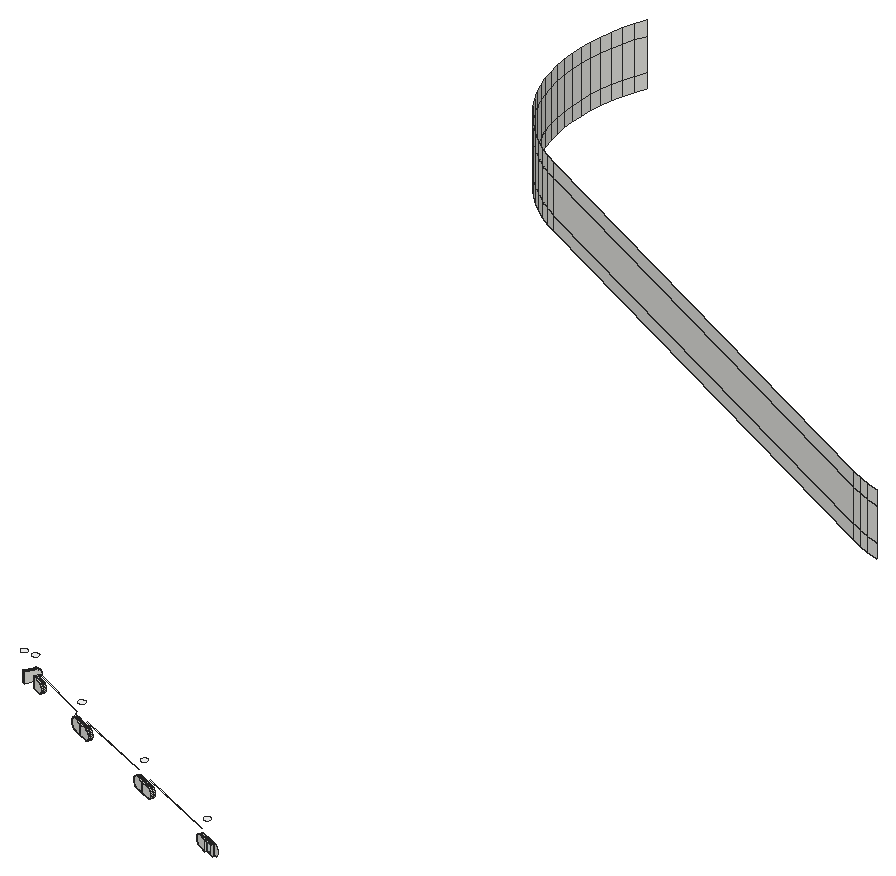
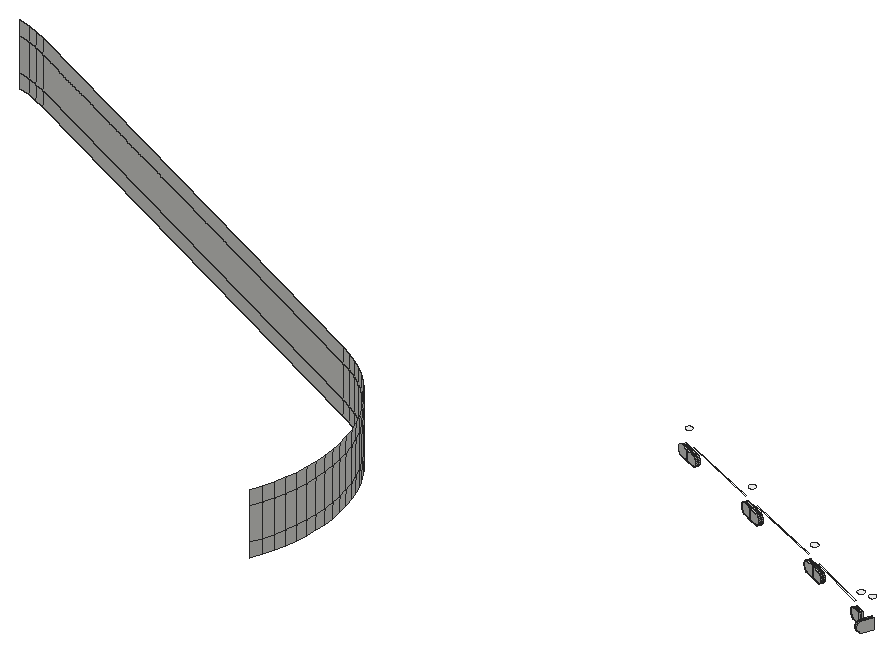
# SketchUp Ruby script. Lengths in inches.
U = 1.inch
M = Sketchup.active_model
def pt(a) = Geom::Point3d.new(a.map { |v| v * U })
def face(e, loops, mat)
  f = e.add_face(loops[0].map { |a| pt(a) })
  loops[1..].each { |l| e.add_face(l.map { |a| pt(a) }).erase! }
  f.material = f.back_material = mat if mat
  f
end
# faces: each face lists its corners as indices into pts; further lists are holes
def faces(e, pts, list, mat = nil) = list.each { |f| face(e, (f[0].is_a?(Array) ? f : [f]).map { |l| l.map { |i| pts[i] } }, mat) }
# xy, xz, yz: faces in a plane at the given z, y or x. An outline is a flat list of corners, or four numbers for a rectangle; further outlines are holes
def ring(l) = l.size == 4 ? [[l[0], l[1]], [l[2], l[1]], [l[2], l[3]], [l[0], l[3]]] : l.each_slice(2).to_a
def flat(e, list, mat, &to3) = list.each { |f| face(e, (f[0].is_a?(Array) ? f : [f]).map { |l| ring(l).map { |u, v| to3.(u, v) } }, mat) }
def xy(e, z, list, mat = nil) = flat(e, list, mat) { |x, y| [x, y, z] }
def xz(e, y, list, mat = nil) = flat(e, list, mat) { |x, z| [x, y, z] }
def yz(e, x, list, mat = nil) = flat(e, list, mat) { |y, z| [x, y, z] }
def lines(e, pts, list) = list.each { |a, b| e.add_line(pt(pts[a]), pt(pts[b])) }
# prism: a flat outline (further loops are holes) pulled along v
def prism(e, loops, v, mat = nil)
  f = face(e, loops, mat); d = Geom::Vector3d.new(v.map { |x| x * U })
  f.pushpull(f.normal.samedirection?(d) ? d.length : -d.length)
end
def box(e, o, s, mat = nil) = prism(e, [[o, [o[0] + s[0], o[1], o[2]], [o[0] + s[0], o[1] + s[1], o[2]], [o[0], o[1] + s[1], o[2]]]], [0, 0, s[2]], mat)
def at(x, y, z, deg = 0) = Geom::Transformation.translation(pt([x, y, z])) * Geom::Transformation.rotation(ORIGIN, Z_AXIS, deg.degrees)
def axes(o, x, y, z) = Geom::Transformation.new([*x, 0, *y, 0, *z, 0, *pt(o).to_a, 1])
def part(name) = M.definitions.add(name)
# library, detail: a bought-in or finely detailed component or shape, given as its bounding box
def library(name, o, s) = part(name).tap { |d| box(d.entities, o, s) }
def detail(e, o, s) = box(e.add_group.entities, o, s)
def put(e, d, t, mat = nil) = e.add_instance(d, t).tap { |i| i.material = mat if mat }
def group(e, t, mat = nil) = e.add_group.tap { |g| g.transformation = t; g.material = mat if mat }.entities
root = M.entities
M.materials.add("Glass_Safety_01").color = [204, 235, 244]
M.materials["Glass_Safety_01"].alpha = 0.1
M.materials.add("[Color_000]").color = [255, 255, 255]
xy(root,351.283,[[614.266,633.854,612.461,634.64,612.571,634.892,614.376,634.106],[612.272,634.207,610.467,634.993,610.577,635.245,610.74,635.174,612.382,634.459],[612.461,634.64,610.819,635.355,610.656,635.426,610.766,635.678,612.571,634.892],[594.081,642.129,592.276,642.915,592.386,643.168,594.191,642.382],[594.27,642.5625,592.465,643.349,592.575,643.601,594.38,642.815],
  [592.276,642.915,590.471,643.701,590.581,643.954,590.746,643.883,592.386,643.168],[592.465,643.349,590.824,644.063,590.66,644.135,590.77,644.387,592.575,643.601],[574.269,650.758,572.464,651.544,572.574,651.797,574.379,651.011],[574.457,651.191,572.656,651.976,572.775,652.224,574.567,651.444],[572.452,651.55,570.677,652.401,570.796,652.65,570.999,652.552,572.571,651.798],
  [572.656,651.976,572.653,651.977,572.763,652.23,572.775,652.224],[572.653,651.977,571.084,652.73,570.881,652.827,571,653.076,572.763,652.23],[558.693,658.15,556.918,659.001,557.037,659.25,558.812,658.398],[558.897,658.576,557.122,659.427,557.241,659.675,559.016,658.824],[555.045,659.23,554.792,659.34,555.578,661.144,555.831,661.034],
  [554.612,659.418,554.359,659.528,555.145,661.333,555.398,661.223]])
xy(root,351.362,[[613.826,633.83,612.382,634.459,612.461,634.64,613.905,634.011],[612.382,634.459,610.938,635.088,611.017,635.269,612.461,634.64],[593.83,642.539,592.386,643.168,592.465,643.349,593.909,642.72],[592.386,643.168,590.942,643.797,591.021,643.977,592.465,643.349],[574.018,651.168,572.574,651.797,572.613,651.887,572.656,651.976,574.096,651.349],
  [572.571,651.798,571.151,652.48,571.236,652.657,572.653,651.977,572.613,651.887],[572.613,651.887,572.653,651.977,572.654,651.977,572.656,651.976],[558.457,658.568,557.037,659.25,557.122,659.427,558.542,658.746],[554.792,659.34,554.612,659.418,555.24,660.862,555.421,660.783]],"Glass_Safety_01")
xy(root,353.33,[[613.826,633.83,613.905,634.011,612.461,634.64,612.382,634.459],[612.382,634.459,612.461,634.64,611.017,635.269,610.938,635.088],[593.83,642.539,593.909,642.72,592.465,643.349,592.386,643.168],[592.386,643.168,592.465,643.349,591.021,643.977,590.942,643.797],[574.018,651.168,574.096,651.349,572.656,651.976,572.613,651.887,572.574,651.797],
  [572.571,651.798,572.613,651.887,572.653,651.977,571.236,652.657,571.151,652.48],[572.613,651.887,572.656,651.976,572.654,651.977,572.653,651.977],[558.457,658.568,558.542,658.746,557.122,659.427,557.037,659.25],[554.792,659.34,555.421,660.783,555.24,660.862,554.612,659.418]],"Glass_Safety_01")
xy(root,353.409,[[614.077,633.421,614.187,633.673,612.382,634.459,612.272,634.207],[614.266,633.854,614.376,634.106,612.571,634.892,612.461,634.64],[612.272,634.207,612.382,634.459,610.74,635.174,610.577,635.245,610.467,634.993],[612.461,634.64,612.571,634.892,610.766,635.678,610.656,635.426,610.819,635.355],[594.081,642.129,594.191,642.382,592.386,643.168,592.276,642.915],
  [594.27,642.5625,594.38,642.815,592.575,643.601,592.465,643.349],[592.276,642.915,592.386,643.168,590.746,643.883,590.581,643.954,590.471,643.701],[592.465,643.349,592.575,643.601,590.77,644.387,590.66,644.135,590.824,644.063],[574.269,650.758,574.379,651.011,572.574,651.797,572.464,651.544],[574.457,651.191,574.567,651.444,572.775,652.224,572.656,651.976],
  [572.452,651.55,572.571,651.798,570.999,652.552,570.796,652.65,570.677,652.401],[572.656,651.976,572.775,652.224,572.763,652.23,572.653,651.977],[572.653,651.977,572.763,652.23,571,653.076,570.881,652.827,571.084,652.73],[558.693,658.15,558.812,658.398,557.037,659.25,556.918,659.001],[558.897,658.576,559.016,658.824,557.241,659.675,557.122,659.427],
  [555.045,659.23,555.831,661.034,555.578,661.144,554.792,659.34],[554.612,659.418,555.398,661.223,555.145,661.333,554.359,659.528]])
xy(root,354.511,[[610.74,635.174,610.819,635.355,594.191,642.382],[610.819,635.355,594.27,642.5625,594.191,642.382],[590.746,643.883,590.824,644.063,574.379,651.011],[590.824,644.063,574.457,651.191,574.379,651.011],[570.999,652.552,571.084,652.73,558.812,658.398],
  [571.084,652.73,558.897,658.576,558.812,658.398]],"Glass_Safety_01")
xy(root,357.267,[[612.467,633.921,612.628,633.954,612.775,634.028,612.898,634.137,612.988,634.274,613.04,634.43,613.05,634.595,613.017,634.756,612.943,634.903,612.834,635.026,612.697,635.116,612.541,635.168,612.376,635.178,612.215,635.145,612.068,635.071,611.945,634.962,611.855,634.825,611.803,634.669,611.793,634.504,611.826,634.343,611.9,634.196,612.009,634.073,612.146,633.983,612.302,633.931],[592.471,642.63,592.632,642.663,592.779,642.737,592.902,642.846,592.992,642.983,593.044,643.139,593.054,643.303,593.021,643.464,592.947,643.612,592.838,643.734,592.701,643.825,592.545,643.877,592.38,643.887,592.219,643.854,592.072,643.78,591.949,643.671,591.859,643.534,591.807,643.377,591.797,643.213,591.83,643.052,591.904,642.905,592.013,642.782,592.15,642.692,592.306,642.64],[572.658,651.259,572.819,651.292,572.966,651.366,573.089,651.475,573.18,651.612,573.232,651.768,573.242,651.932,573.209,652.093,573.135,652.24,573.026,652.363,572.888,652.454,572.732,652.506,572.568,652.515,572.407,652.482,572.26,652.409,572.137,652.3,572.047,652.162,571.995,652.006,571.985,651.842,572.018,651.681,572.092,651.534,572.201,651.411,572.338,651.321,572.494,651.269],[557.124,658.71,557.286,658.743,557.433,658.817,557.556,658.926,557.646,659.063,557.698,659.219,557.708,659.383,557.675,659.544,557.601,659.691,557.492,659.814,557.355,659.905,557.199,659.957,557.034,659.967,556.873,659.933,556.726,659.86,556.603,659.751,556.513,659.613,556.461,659.457,556.451,659.293,556.484,659.132,556.558,658.985,556.667,658.862,556.804,658.772,556.96,658.72],[554.747,658.751,554.908,658.784,555.055,658.857,555.178,658.966,555.268,659.104,555.32,659.26,555.33,659.424,555.297,659.585,555.223,659.732,555.114,659.855,554.977,659.946,554.821,659.997,554.657,660.007,554.496,659.974,554.349,659.901,554.226,659.791,554.135,659.654,554.083,659.498,554.073,659.334,554.107,659.173,554.18,659.026,554.289,658.903,554.427,658.812,554.583,658.76]],"[Color_000]")
p = [[612.382,634.459,353.409],[614.187,633.673,353.409],[614.187,633.673,351.283],[612.382,634.459,351.283],[612.382,634.459,351.362],[613.826,633.83,351.362],
  [613.826,633.83,353.33],[612.382,634.459,353.33],[612.571,634.892,353.409],[614.376,634.106,353.409],[614.628,633.997,353.373],[614.863,633.894,353.267],
  [615.065,633.806,353.098],[615.22,633.739,352.877],[615.317,633.696,352.621],[615.35,633.682,352.346],[615.317,633.696,352.071],[615.22,633.739,351.815],
  [615.065,633.806,351.594],[614.863,633.894,351.425],[614.628,633.997,351.319],[614.376,634.106,351.283],[612.571,634.892,351.283],[612.461,634.64,351.283],
  [614.266,633.854,351.283],[614.266,633.854,353.409],[612.461,634.64,353.409],[612.461,634.64,353.33],[613.905,634.011,353.33],[613.905,634.011,351.362],
  [612.461,634.64,351.362],[612.272,634.207,353.409],[610.467,634.993,353.409],[610.215,635.102,353.373],[609.98,635.205,353.267],[609.778,635.293,353.098],
  [609.623,635.36,352.877],[609.526,635.403,352.621],[609.493,635.417,352.346],[609.526,635.403,352.071],[609.623,635.36,351.815],[609.778,635.293,351.594],
  [609.98,635.205,351.425],[610.215,635.102,351.319],[610.467,634.993,351.283],[612.272,634.207,351.283],[610.74,635.174,351.283],[610.74,635.174,353.409],
  [610.938,635.088,353.33],[610.938,635.088,351.362],[610.819,635.355,353.409],[610.819,635.355,351.283],[611.017,635.269,351.362],[611.017,635.269,353.33],
  [610.766,635.678,353.409],[610.766,635.678,351.283],[610.514,635.788,351.319],[610.279,635.891,351.425],[610.077,635.979,351.594],[609.922,636.046,351.815],
  [609.825,636.088,352.071],[609.792,636.103,352.346],[609.825,636.088,352.621],[609.922,636.046,352.877],[610.077,635.979,353.098],[610.279,635.891,353.267],
  [610.514,635.788,353.373],[610.325,635.355,351.319],[610.577,635.245,351.283],[610.09,635.458,351.425],[610.577,635.245,353.409],[609.888,635.545,351.594],
  [609.733,635.613,351.815],[609.636,635.655,352.071],[609.603,635.67,352.346],[609.636,635.655,352.621],[609.733,635.613,352.877],[609.888,635.545,353.098],
  [610.09,635.458,353.267],[610.325,635.355,353.373],[610.656,635.426,351.283],[610.656,635.426,353.409],[610.404,635.536,353.373],[610.169,635.638,353.267],
  [609.967,635.726,353.098],[609.812,635.793,352.877],[609.715,635.836,352.621],[609.681,635.85,352.346],[609.715,635.836,352.071],[609.812,635.793,351.815],
  [609.967,635.726,351.594],[610.169,635.638,351.425],[610.404,635.536,351.319],[594.081,642.129,353.409],[592.276,642.915,353.409],[592.276,642.915,351.283],
  [594.081,642.129,351.283],[594.333,642.02,351.319],[594.568,641.917,351.425],[594.77,641.829,351.594],[594.925,641.762,351.815],[595.022,641.719,352.071],
  [595.056,641.705,352.346],[595.022,641.719,352.621],[594.925,641.762,352.877],[594.77,641.829,353.098],[594.568,641.917,353.267],[594.333,642.02,353.373],
  [594.443,642.272,351.319],[594.678,642.17,351.425],[594.191,642.382,351.283],[594.191,642.382,353.409],[594.88,642.082,351.594],[595.035,642.014,351.815],
  [595.132,641.972,352.071],[595.166,641.958,352.346],[595.132,641.972,352.621],[595.035,642.014,352.877],[594.88,642.082,353.098],[594.678,642.17,353.267],
  [594.443,642.272,353.373],[594.27,642.5625,351.283],[594.27,642.5625,353.409],[594.522,642.453,353.373],[594.757,642.35,353.267],[594.959,642.262,353.098],
  [595.114,642.195,352.877],[595.211,642.153,352.621],[595.244,642.138,352.346],[595.211,642.153,352.071],[595.114,642.195,351.815],[594.959,642.262,351.594],
  [594.757,642.35,351.425],[594.522,642.453,351.319],[592.386,643.168,353.409],[592.386,643.168,351.283],[592.386,643.168,351.362],[593.83,642.539,351.362],
  [593.83,642.539,353.33],[592.386,643.168,353.33],[592.575,643.601,353.409],[594.38,642.815,353.409],[594.632,642.705,353.373],[594.867,642.603,353.267],
  [595.069,642.515,353.098],[595.224,642.448,352.877],[595.321,642.405,352.621],[595.354,642.391,352.346],[595.321,642.405,352.071],[595.224,642.448,351.815],
  [595.069,642.515,351.594],[594.867,642.603,351.425],[594.632,642.705,351.319],[594.38,642.815,351.283],[592.575,643.601,351.283],[592.465,643.349,351.283],
  [592.465,643.349,353.409],[592.465,643.349,353.33],[593.909,642.72,353.33],[593.909,642.72,351.362],[592.465,643.349,351.362],[590.471,643.701,353.409],
  [590.219,643.811,353.373],[589.984,643.914,353.267],[589.782,644.002,353.098],[589.627,644.069,352.877],[589.53,644.111,352.621],[589.497,644.126,352.346],
  [589.53,644.111,352.071],[589.627,644.069,351.815],[589.782,644.002,351.594],[589.984,643.914,351.425],[590.219,643.811,351.319],[590.471,643.701,351.283],
  [590.746,643.883,351.283],[590.746,643.883,353.409],[590.942,643.797,353.33],[590.942,643.797,351.362],[590.824,644.063,353.409],[590.824,644.063,351.283],
  [591.021,643.977,351.362],[591.021,643.977,353.33],[590.77,644.387,353.409],[590.77,644.387,351.283],[590.518,644.497,351.319],[590.283,644.6,351.425],
  [590.081,644.6875,351.594],[589.926,644.755,351.815],[589.829,644.797,352.071],[589.796,644.812,352.346],[589.829,644.797,352.621],[589.926,644.755,352.877],
  [590.081,644.6875,353.098],[590.283,644.6,353.267],[590.518,644.497,353.373],[590.329,644.064,351.319],[590.581,643.954,351.283],[590.094,644.166,351.425],
  [590.581,643.954,353.409],[589.892,644.254,351.594],[589.737,644.322,351.815],[589.64,644.364,352.071],[589.607,644.379,352.346],[589.64,644.364,352.621],
  [589.737,644.322,352.877],[589.892,644.254,353.098],[590.094,644.166,353.267],[590.329,644.064,353.373],[590.66,644.135,351.283],[590.66,644.135,353.409],
  [590.408,644.244,353.373],[590.173,644.347,353.267],[589.971,644.435,353.098],[589.816,644.502,352.877],[589.719,644.545,352.621],[589.685,644.559,352.346],
  [589.719,644.545,352.071],[589.816,644.502,351.815],[589.971,644.435,351.594],[590.173,644.347,351.425],[590.408,644.244,351.319],[574.269,650.758,353.409],
  [572.464,651.544,353.409],[572.464,651.544,351.283],[574.269,650.758,351.283],[574.521,650.648,351.319],[574.756,650.546,351.425],[574.958,650.458,351.594],
  [575.113,650.391,351.815],[575.21,650.348,352.071],[575.243,650.334,352.346],[575.21,650.348,352.621],[575.113,650.391,352.877],[574.958,650.458,353.098],
  [574.756,650.546,353.267],[574.521,650.648,353.373],[574.631,650.901,351.319],[574.866,650.799,351.425],[574.379,651.011,351.283],[574.379,651.011,353.409],
  [575.068,650.711,351.594],[575.223,650.643,351.815],[575.32,650.601,352.071],[575.353,650.586,352.346],[575.32,650.601,352.621],[575.223,650.643,352.877],
  [575.068,650.711,353.098],[574.866,650.799,353.267],[574.631,650.901,353.373],[574.457,651.191,353.409],[572.656,651.976,353.409],[572.656,651.976,353.33],
  [574.096,651.349,353.33],[574.096,651.349,351.362],[572.656,651.976,351.362],[572.656,651.976,351.283],[574.457,651.191,351.283],[574.71,651.082,351.319],
  [574.945,650.979,351.425],[575.147,650.891,351.594],[575.301,650.824,351.815],[575.399,650.781,352.071],[575.432,650.767,352.346],[575.399,650.781,352.621],
  [575.301,650.824,352.877],[575.147,650.891,353.098],[574.945,650.979,353.267],[574.71,651.082,353.373],[572.574,651.797,353.409],[572.574,651.797,351.283],
  [572.574,651.797,351.362],[574.018,651.168,351.362],[574.018,651.168,353.33],[572.574,651.797,353.33],[572.763,652.23,353.409],[572.769,652.227,353.409],
  [572.775,652.224,353.409],[574.567,651.444,353.409],[574.82,651.334,353.373],[575.055,651.232,353.267],[575.257,651.144,353.098],[575.411,651.076,352.877],
  [575.509,651.034,352.621],[575.542,651.02,352.346],[575.509,651.034,352.071],[575.411,651.076,351.815],[575.257,651.144,351.594],[575.055,651.232,351.425],
  [574.82,651.334,351.319],[574.567,651.444,351.283],[572.775,652.224,351.283],[572.769,652.227,351.283],[572.763,652.23,351.283],[572.452,651.55,353.409],
  [570.677,652.401,353.409],[570.429,652.52,353.373],[570.197,652.631,353.267],[569.999,652.726,353.098],[569.847,652.799,352.877],[569.751,652.845,352.621],
  [569.718,652.861,352.346],[569.751,652.845,352.071],[569.847,652.799,351.815],[569.999,652.726,351.594],[570.197,652.631,351.425],[570.429,652.52,351.319],
  [570.677,652.401,351.283],[572.452,651.55,351.283],[572.571,651.798,351.283],[572.571,651.798,351.362],[572.571,651.798,353.33],[572.571,651.798,353.409],
  [570.999,652.552,351.283],[570.999,652.552,353.409],[571.151,652.48,353.33],[571.151,652.48,351.362],[572.653,651.977,351.283],[572.653,651.977,351.362],
  [571.236,652.657,351.362],[571.236,652.657,353.33],[572.653,651.977,353.33],[572.653,651.977,353.409],[571.084,652.73,353.409],[571.084,652.73,351.283],
  [572.654,651.977,351.362],[571,653.076,353.409],[571,653.076,351.283],[570.752,653.195,351.319],[570.521,653.306,351.425],[570.322,653.401,351.594],
  [570.17,653.474,351.815],[570.074,653.52,352.071],[570.042,653.535,352.346],[570.074,653.52,352.621],[570.17,653.474,352.877],[570.322,653.401,353.098],
  [570.521,653.306,353.267],[570.752,653.195,353.373],[570.548,652.769,351.319],[570.796,652.65,351.283],[570.317,652.88,351.425],[570.118,652.975,351.594],
  [569.966,653.048,351.815],[569.87,653.094,352.071],[569.837,653.11,352.346],[569.839,653.109,352.36],[570.332,652.873,353.273],[570.548,652.769,353.373],
  [570.796,652.65,353.409],[570.881,652.827,351.283],[570.881,652.827,353.409],[570.633,652.946,353.373],[570.402,653.057,353.267],[570.203,653.152,353.098],
  [570.051,653.225,352.877],[569.955,653.271,352.621],[569.923,653.287,352.346],[569.955,653.271,352.071],[570.051,653.225,351.815],[570.203,653.152,351.594],
  [570.402,653.057,351.425],[570.633,652.946,351.319],[558.693,658.15,353.409],[556.918,659.001,353.409],[556.918,659.001,351.283],[558.693,658.15,351.283],
  [558.941,658.031,351.319],[559.172,657.92,351.425],[559.37,657.825,351.594],[559.523,657.752,351.815],[559.618,657.706,352.071],[559.651,657.69,352.346],
  [559.618,657.706,352.621],[559.523,657.752,352.877],[559.37,657.825,353.098],[559.172,657.92,353.267],[558.941,658.031,353.373],[558.812,658.398,353.409],
  [558.812,658.398,351.283],[559.06,658.279,351.319],[559.291,658.168,351.425],[559.489,658.073,351.594],[559.642,658,351.815],[559.738,657.954,352.071],
  [559.77,657.938,352.346],[559.738,657.954,352.621],[559.642,658,352.877],[559.489,658.073,353.098],[559.291,658.168,353.267],[559.06,658.279,353.373],
  [558.897,658.576,351.283],[558.897,658.576,353.409],[559.145,658.457,353.373],[559.376,658.346,353.267],[559.575,658.251,353.098],[559.727,658.178,352.877],
  [559.823,658.132,352.621],[559.855,658.116,352.346],[559.823,658.132,352.071],[559.727,658.178,351.815],[559.575,658.251,351.594],[559.376,658.346,351.425],
  [559.145,658.457,351.319],[559.264,658.705,351.319],[559.495,658.594,351.425],[557.037,659.25,353.409],[557.037,659.25,351.283],[557.037,659.25,351.362],
  [558.457,658.568,351.362],[558.457,658.568,353.33],[557.037,659.25,353.33],[557.241,659.675,353.409],[559.016,658.824,353.409],[559.264,658.705,353.373],
  [559.495,658.594,353.267],[559.694,658.499,353.098],[559.846,658.426,352.877],[559.942,658.38,352.621],[559.975,658.364,352.346],[559.942,658.38,352.071],
  [559.846,658.426,351.815],[559.694,658.499,351.594],[559.016,658.824,351.283],[557.241,659.675,351.283],[557.122,659.427,351.283],[557.122,659.427,353.409],
  [557.122,659.427,353.33],[558.542,658.746,353.33],[558.542,658.746,351.362],[557.122,659.427,351.362],[554.792,659.34,351.362],[554.792,659.34,351.283],
  [555.045,659.23,351.283],[555.045,659.23,353.409],[554.792,659.34,353.409],[554.792,659.34,353.33],[555.831,661.034,353.409],[555.831,661.034,351.283],
  [555.941,661.287,351.319],[556.043,661.522,351.425],[556.131,661.723,351.594],[556.198,661.878,351.815],[556.241,661.976,352.071],[556.255,662.009,352.346],
  [556.241,661.976,352.621],[556.198,661.878,352.877],[556.131,661.723,353.098],[556.043,661.522,353.267],[555.941,661.287,353.373],[555.578,661.144,353.409],
  [555.688,661.397,353.373],[555.79,661.632,353.267],[555.878,661.834,353.098],[555.946,661.988,352.877],[555.988,662.086,352.621],[556.002,662.119,352.346],
  [555.988,662.086,352.071],[555.946,661.988,351.815],[555.878,661.834,351.594],[555.79,661.632,351.425],[555.688,661.397,351.319],[555.578,661.144,351.283],
  [555.421,660.783,351.362],[555.421,660.783,353.33],[554.612,659.418,351.283],[554.612,659.418,351.362],[554.612,659.418,353.33],[554.612,659.418,353.409],
  [554.359,659.528,353.409],[554.359,659.528,351.283],[555.398,661.223,353.409],[555.24,660.862,353.33],[555.24,660.862,351.362],[555.398,661.223,351.283],
  [555.507,661.475,351.319],[555.61,661.71,351.425],[555.698,661.912,351.594],[555.765,662.067,351.815],[555.808,662.164,352.071],[555.822,662.198,352.346],
  [555.808,662.164,352.621],[555.765,662.067,352.877],[555.698,661.912,353.098],[555.61,661.71,353.267],[555.507,661.475,353.373],[555.145,661.333,353.409],
  [555.255,661.585,353.373],[555.357,661.82,353.267],[555.445,662.022,353.098],[555.512,662.177,352.877],[555.555,662.274,352.621],[555.569,662.308,352.346],
  [555.555,662.274,352.071],[555.512,662.177,351.815],[555.445,662.022,351.594],[555.357,661.82,351.425],[555.255,661.585,351.319],[555.145,661.333,351.283],
  [572.613,651.887,353.33],[572.613,651.887,351.362],[572.654,651.977,353.33],[569.87,653.094,352.621],[569.966,653.048,352.877],[570.118,652.975,353.098],
  [570.317,652.88,353.267],[570.999,652.552,354.511],[702.697,692.459,415.758],[702.697,692.459,412.837],[704.956,691.789,412.837],[704.956,691.789,415.758],
  [700.488,693.275,415.758],[700.488,693.275,412.837],[698.336,694.234,415.758],[698.336,694.234,412.837],[596.965,743.457,415.758],[596.965,743.457,412.837],
  [594.881,744.555,415.758],[594.881,744.555,412.837],[592.872,745.787,415.758],[592.872,745.787,412.837],[590.949,747.147,415.758],[590.949,747.147,412.837],
  [589.119,748.631,415.758],[589.119,748.631,412.837],[587.39,750.231,415.758],[587.39,750.231,412.837],[585.769,751.94,415.758],[585.769,751.94,412.837],
  [584.263,753.752,415.758],[584.263,753.752,412.837],[582.88,755.658,415.758],[582.88,755.658,412.837],[581.623,757.651,415.758],[581.623,757.651,412.837],
  [580.5,759.722,415.758],[580.5,759.722,412.837],[579.515,761.862,415.758],[579.515,761.862,412.837],[578.672,764.062,415.758],[578.672,764.062,412.837],
  [577.974,766.312,415.758],[577.974,766.312,412.837],[577.425,768.603,415.758],[577.425,768.603,412.837],[577.027,770.924,415.758],[577.027,770.924,412.837],
  [576.782,773.267,415.758],[576.782,773.267,412.837],[576.69,775.621,415.758],[576.69,775.621,412.837],[576.753,777.976,415.758],[576.753,777.976,412.837],
  [576.97,780.322,415.758],[576.97,780.322,412.837],[577.339,782.649,415.758],[577.339,782.649,412.837],[577.86,784.946,415.758],[577.86,784.946,412.837],
  [578.53,787.205,415.758],[578.53,787.205,412.837],[579.347,789.415,415.758],[579.347,789.415,412.837],[704.956,691.789,422.51],[702.697,692.459,422.51],
  [700.488,693.275,422.51],[698.336,694.234,422.51],[596.965,743.457,422.51],[594.881,744.555,422.51],[592.872,745.787,422.51],[590.949,747.147,422.51],
  [589.119,748.631,422.51],[587.39,750.231,422.51],[585.769,751.94,422.51],[584.263,753.752,422.51],[582.88,755.658,422.51],[581.623,757.651,422.51],
  [580.5,759.722,422.51],[579.515,761.862,422.51],[578.672,764.062,422.51],[577.974,766.312,422.51],[577.425,768.603,422.51],[577.027,770.924,422.51],
  [576.782,773.267,422.51],[576.69,775.621,422.51],[576.753,777.976,422.51],[576.97,780.322,422.51],[577.339,782.649,422.51],[577.86,784.946,422.51],
  [578.53,787.205,422.51],[579.347,789.415,422.51],[704.956,691.789,425.526],[702.697,692.459,425.526],[700.488,693.275,425.526],[698.336,694.234,425.526],
  [596.965,743.457,425.526],[594.881,744.555,425.526],[592.872,745.787,425.526],[590.949,747.147,425.526],[589.119,748.631,425.526],[587.39,750.231,425.526],
  [585.769,751.94,425.526],[584.263,753.752,425.526],[582.88,755.658,425.526],[581.623,757.651,425.526],[580.5,759.722,425.526],[579.515,761.862,425.526],
  [578.672,764.062,425.526],[577.974,766.312,425.526],[577.425,768.603,425.526],[577.027,770.924,425.526],[576.782,773.267,425.526],[576.69,775.621,425.526],
  [576.753,777.976,425.526],[576.97,780.322,425.526],[577.339,782.649,425.526],[577.86,784.946,425.526],[578.53,787.205,425.526],[579.347,789.415,425.526]]
faces(root,p,[[0,1,2,3,4,5,6,7],[8,9,10,11,12,13,14,15,16,17,18,19,20,21,22],[23,24,25,26,27,28,29,30],[31,32,33,34,35,36,37,38,39,40,41,42,43,44,45],[3,4,7,0,31,45],[3,46,47,0,7,48,49,4],[26,50,51,23,30,52,53,27],[30,23,22,8,26,27],
  [54,8,22,55,56,57,58,59,60,61,62,63,64,65,66],[67,68,44,43],[69,67,43,42],[70,47,46,68,67,69,71,72,73,74,75,76,77,78,79],[80,51,50,81,82,83,84,85,86,87,88,89,90,91,92],[80,92,56,55],[92,91,57,56],[93,94,95,96,97,98,99,100,101,102,103,104,105,106,107],
  [108,109,98,97],[110,108,97,96],[134,111,110,135,136,137,138,139],[140,141,142,143,144,145,146,147,148,149,150,151,152,153,154],[132,133,152,151],[133,121,153,152],[155,121,122,156,157,158,159,160],[94,161,162,163,164,165,166,167,168,169,170,171,172,173,95],
  [135,136,139,134,94,95],[135,174,175,134,139,176,177,136],[156,178,179,155,160,180,181,157],[160,155,154,140,156,157],[182,140,154,183,184,185,186,187,188,189,190,191,192,193,194],[195,196,173,172],[197,195,172,171],[198,175,174,196,195,197,199,200,201,202,203,204,205,206,207],
  [208,179,178,209,210,211,212,213,214,215,216,217,218,219,220],[208,220,184,183],[220,219,185,184],[221,222,223,224,225,226,227,228,229,230,231,232,233,234,235],[236,237,226,225],[238,236,225,224],[249,250,251,252,253,254,255,256,257,258,259,260,261,262,263,264,265,266,267],[268,239,238,269,270,271,272,273],
  [274,275,276,277,278,279,280,281,282,283,284,285,286,287,288,289,290,291,292],[258,257,288,287],[257,256,289,288],[293,294,295,296,297,298,299,300,301,302,303,304,305,306,307],[270,269,223,222,268,273],[308,309,310,311,293,307],[308,312,313,311,310,314,315,309],[316,317,318,319,320,321,322,323],
  [250,321,320,317,316,255,254,251],[316,255,254,324,317],[254,255,290,276,250,251],[316,317,320,321,274,292],[325,274,292,326,327,328,329,330,331,332,333,334,335,336,337],[291,292,274,275,276,290],[338,339,306,305],[340,338,305,304],
  [349,323,322,350,351,352,353,354,355,356,357,358,359,360,361],[349,361,327,326],[361,360,328,327],[362,363,364,365,366,367,368,369,370,371,372,373,374,375,376],[379,380,367,366],[378,379,366,365],[401,402,403,404],[405,377,378,406,407,408,409,410],
  [411,412,413,414,415,416,417,418,419,420,421,404,403,422,423],[402,390,422,403],[424,390,391,425,426,427,428,429],[407,406,364,363,405,410],[430,431,432,433,434,435],[436,433,432,437,438,439,440,441,442,443,444,445,446,447,448],[434,449,450,451,452,453,454,455,456,457,458,459,460,461,431,430,462,463,435],[464,465,466,467,468,469],
  [470,467,466,471,472,465,464,473,474,475,476,477,478,479,480,481,482,483,484],[424,429,426,425,411,423],[468,485,486,487,488,489,490,491,492,493,494,495,496,497,469],[461,460,438,437],[474,473,497,496],[460,459,439,438],[475,474,496,495],[71,69,42,41],
  [91,90,58,57],[109,112,99,98],[131,132,151,150],[199,197,171,170],[219,218,186,185],[237,240,227,226],[259,258,287,286],[341,340,304,303],
  [360,359,329,328],[380,381,368,367],[400,401,404,421],[459,458,440,439],[476,475,495,494],[72,71,41,40],[90,89,59,58],[112,113,100,99],
  [130,131,150,149],[200,199,170,169],[218,217,187,186],[240,241,228,227],[260,259,286,285],[342,341,303,302],[359,358,330,329],[381,382,369,368],
  [399,400,421,420],[458,457,441,440],[477,476,494,493],[73,72,40,39],[89,88,60,59],[113,114,101,100],[129,130,149,148],[201,200,169,168],
  [217,216,188,187],[241,242,229,228],[261,260,285,284],[343,342,302,301],[358,357,331,330],[382,383,370,369],[398,399,420,419],[457,456,442,441],
  [478,477,493,492],[74,73,39,38],[88,87,61,60],[114,115,102,101],[128,129,148,147],[202,201,168,167],[216,215,189,188],[242,243,230,229],
  [262,261,284,283],[344,343,301,300],[357,356,332,331],[383,384,371,370],[397,398,419,418],[456,455,443,442],[479,478,492,491],[75,74,38,37],
  [87,86,62,61],[115,116,103,102],[127,128,147,146],[203,202,167,166],[215,214,190,189],[243,244,231,230],[263,262,283,282],[501,345,344,300,299],
  [356,355,333,332],[384,385,372,371],[396,397,418,417],[455,454,444,443],[480,479,491,490],[345,501,502,503,504,346],[76,75,37,36],[86,85,63,62],
  [116,117,104,103],[126,127,146,145],[204,203,166,165],[214,213,191,190],[244,245,232,231],[264,263,282,281],[502,501,299,298],[355,354,334,333],
  [385,386,373,372],[395,396,417,416],[454,453,445,444],[481,480,490,489],[77,76,36,35],[85,84,64,63],[117,118,105,104],[125,126,145,144],
  [205,204,165,164],[213,212,192,191],[245,246,233,232],[265,264,281,280],[503,502,298,297],[354,353,335,334],[386,387,374,373],[394,395,416,415],
  [453,452,446,445],[482,481,489,488],[78,77,35,34],[84,83,65,64],[118,119,106,105],[124,125,144,143],[206,205,164,163],[212,211,193,192],
  [246,247,234,233],[266,265,280,279],[504,503,297,296],[353,352,336,335],[387,388,375,374],[393,394,415,414],[452,451,447,446],[483,482,488,487],
  [79,78,34,33],[83,82,66,65],[119,120,107,106],[123,124,143,142],[207,206,163,162],[211,210,194,193],[247,248,235,234],[267,266,279,278],
  [500,251,250,321,320],[347,346,504,296,295],[352,351,337,336],[388,389,376,375],[392,393,414,413],[451,450,448,447],[484,483,487,486],[70,79,33,32],
  [82,81,54,66],[120,111,93,107],[122,123,142,141],[198,207,162,161],[210,209,182,194],[248,239,221,235],[249,267,278,277],[348,347,295,294],
  [351,350,325,337],[389,377,362,376],[391,392,413,412],[450,449,436,448],[470,484,486,485],[506,507,508,509],[510,511,507,506],[512,513,511,510],
  [512,514,515,513],[516,517,515,514],[518,519,517,516],[520,521,519,518],[522,523,521,520],[524,525,523,522],[526,527,525,524],[528,529,527,526],
  [530,531,529,528],[532,533,531,530],[534,535,533,532],[536,537,535,534],[538,539,537,536],[540,541,539,538],[542,543,541,540],[544,545,543,542],
  [546,547,545,544],[548,549,547,546],[550,551,549,548],[552,553,551,550],[554,555,553,552],[556,557,555,554],[558,559,557,556],[560,561,559,558],
  [506,509,562,563],[510,506,563,564],[512,510,564,565],[514,512,565,566],[516,514,566,567],[518,516,567,568],[520,518,568,569],[522,520,569,570],
  [524,522,570,571],[526,524,571,572],[528,526,572,573],[530,528,573,574],[532,530,574,575],[534,532,575,576],[536,534,576,577],[538,536,577,578],
  [540,538,578,579],[542,540,579,580],[544,542,580,581],[546,544,581,582],[548,546,582,583],[550,548,583,584],[552,550,584,585],[554,552,585,586],
  [556,554,586,587],[558,556,587,588],[560,558,588,589],[563,562,590,591],[564,563,591,592],[565,564,592,593],[566,565,593,594],[567,566,594,595],
  [568,567,595,596],[569,568,596,597],[570,569,597,598],[571,570,598,599],[572,571,599,600],[573,572,600,601],[574,573,601,602],[575,574,602,603],
  [576,575,603,604],[577,576,604,605],[578,577,605,606],[579,578,606,607],[580,579,607,608],[581,580,608,609],[582,581,609,610],[583,582,610,611],
  [584,583,611,612],[585,584,612,613],[586,585,613,614],[587,586,614,615],[588,587,615,616],[589,588,616,617]])
faces(root,p,[[111,110,108,109,112,113,114,115,116,117,118,119,120],[121,122,123,124,125,126,127,128,129,130,131,132,133],[239,238,236,237,240,241,242,243,244,245,246,247,248],[256,249,267,266,265,264,263,262,261,260,259,258,257],[313,312,339,338,340,341,342,343,344,345,346,347,348],[377,378,379,380,381,382,383,384,385,386,387,388,389],[390,391,392,393,394,395,396,397,398,399,400,401,402],[7,6,5,4],
  [28,27,30,29],[48,7,4,49],[27,7,4,30],[27,53,52,30],[53,52,49,48],[139,138,137,136],[138,137,159,158],[158,157,160,159],
  [176,139,136,177],[157,139,136,160],[157,181,180,160],[181,180,177,176],[273,272,271,270],[271,253,252,272],[252,251,254,253],[314,310,309,315],
  [498,499,270,273],[309,499,498,310],[251,498,499,254],[499,498,320,317],[319,320,317,318],[324,254,251,500,320,317],[319,318,315,314],[410,409,408,407],
  [409,408,428,427],[427,426,429,428],[407,410,426,429],[430,435,466,465],[435,463,462,430],[471,466,465,472],[463,462,472,471],[505,346,347,348,313]],"Glass_Safety_01")
